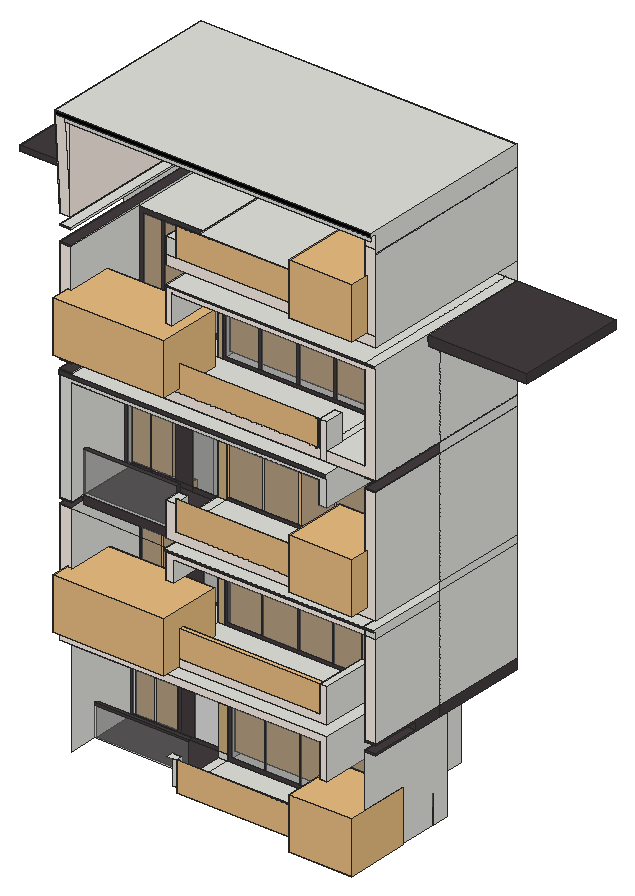
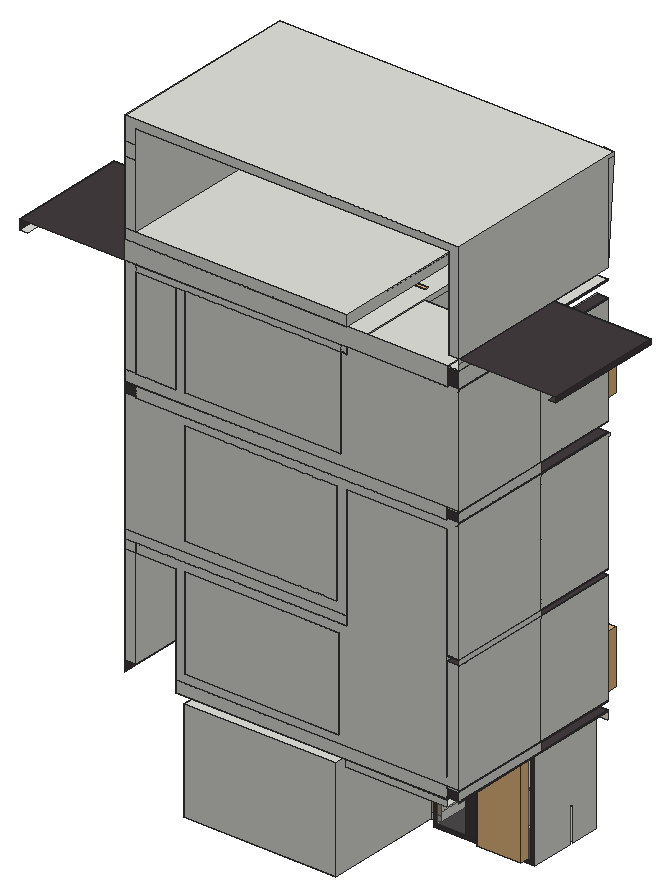
# SketchUp Ruby script. Lengths in inches.
U = 1.inch
M = Sketchup.active_model
def pt(a) = Geom::Point3d.new(a.map { |v| v * U })
def face(e, loops, mat)
  f = e.add_face(loops[0].map { |a| pt(a) })
  loops[1..].each { |l| e.add_face(l.map { |a| pt(a) }).erase! }
  f.material = f.back_material = mat if mat
  f
end
# faces: each face lists its corners as indices into pts; further lists are holes
def faces(e, pts, list, mat = nil) = list.each { |f| face(e, (f[0].is_a?(Array) ? f : [f]).map { |l| l.map { |i| pts[i] } }, mat) }
# xy, xz, yz: faces in a plane at the given z, y or x. An outline is a flat list of corners, or four numbers for a rectangle; further outlines are holes
def ring(l) = l.size == 4 ? [[l[0], l[1]], [l[2], l[1]], [l[2], l[3]], [l[0], l[3]]] : l.each_slice(2).to_a
def flat(e, list, mat, &to3) = list.each { |f| face(e, (f[0].is_a?(Array) ? f : [f]).map { |l| ring(l).map { |u, v| to3.(u, v) } }, mat) }
def xy(e, z, list, mat = nil) = flat(e, list, mat) { |x, y| [x, y, z] }
def xz(e, y, list, mat = nil) = flat(e, list, mat) { |x, z| [x, y, z] }
def yz(e, x, list, mat = nil) = flat(e, list, mat) { |y, z| [x, y, z] }
def lines(e, pts, list) = list.each { |a, b| e.add_line(pt(pts[a]), pt(pts[b])) }
# prism: a flat outline (further loops are holes) pulled along v
def prism(e, loops, v, mat = nil)
  f = face(e, loops, mat); d = Geom::Vector3d.new(v.map { |x| x * U })
  f.pushpull(f.normal.samedirection?(d) ? d.length : -d.length)
end
def box(e, o, s, mat = nil) = prism(e, [[o, [o[0] + s[0], o[1], o[2]], [o[0] + s[0], o[1] + s[1], o[2]], [o[0], o[1] + s[1], o[2]]]], [0, 0, s[2]], mat)
def at(x, y, z, deg = 0) = Geom::Transformation.translation(pt([x, y, z])) * Geom::Transformation.rotation(ORIGIN, Z_AXIS, deg.degrees)
def axes(o, x, y, z) = Geom::Transformation.new([*x, 0, *y, 0, *z, 0, *pt(o).to_a, 1])
def part(name) = M.definitions.add(name)
# library, detail: a bought-in or finely detailed component or shape, given as its bounding box
def library(name, o, s) = part(name).tap { |d| box(d.entities, o, s) }
def detail(e, o, s) = box(e.add_group.entities, o, s)
def put(e, d, t, mat = nil) = e.add_instance(d, t).tap { |i| i.material = mat if mat }
def group(e, t, mat = nil) = e.add_group.tap { |g| g.transformation = t; g.material = mat if mat }.entities
root = M.entities
M.materials.add("Material metal").color = [2, 2, 2]
M.materials.add("[0009_Linen]").color = [250, 240, 230]
M.materials.add("[Asphalt New]").color = [67, 60, 62]
M.materials.add("[Translucent Glass Gray]").color = [128, 128, 128]
M.materials["[Translucent Glass Gray]"].alpha = 0.5
M.materials.add("[Wood Floor Light]").color = [204, 176, 127]
c1 = library("Air Grill2",[0,0,0],[0.79,39.37,4.92])
c2 = library("Planted wooden trough",[0,0,0],[56.02,15.3,25.28])
c3 = library("fronceur+aubin+blanc+(3)",[-47.99,-0.29,1.66],[95.37,4.84,114.09])
xy(root,484.875,[[453.2,361.55,453.47,370.26],[453.47,361.55,628.99,361.55,628.99,440.43,453.2,440.43,453.2,370.26,453.47,370.26],[628.99,361.55,637.96,440.43],[637.96,361.55,684.21,463.55],[441.67,370.26,453.2,440.43],
  [453.2,440.43,628.99,577.24],[637.96,466.33,684.21,486.68]])
xy(root,484.875,[[325.03,399.42,441.42,450.18]],"[Asphalt New]")
xy(root,519.75,[[637.96,463.55,684.21,466.33]])
xy(root,520.45,[[441.67,361.55,453.2,370.26]])
xy(root,524.4375,[[325.03,394.93,441.42,399.42]],"[Asphalt New]")
xy(root,561.74,[[628.99,361.55,637.96,440.43]])
xy(root,602.15,[[325.03,361.55,325.03,519.74,325.23,519.74,325.23,577.24,441.67,577.24,441.67,440.43,628.99,440.43,628.99,361.55],[453.2,440.43,628.99,577.24]])
xy(root,609.74,[[325.03,450.18,441.42,577.24]])
xy(root,610.74,[[325.03,361.55,637.96,577.24]])
xy(root,610.74,[[637.96,422.24,684.21,486.68]],"[Asphalt New]")
xy(root,612.69,[[310.35,361.55,325.03,577.24]],"[Asphalt New]")
xy(root,612.78,[[684.21,361.55,697.64,422.24]],"[Asphalt New]")
xy(root,621.73,[[310.35,361.55,325.03,577.24]],"[Asphalt New]")
xy(root,622.21,[[684.21,361.55,697.64,422.24]],"[Asphalt New]")
xy(root,623.86,[[325.03,361.55,637.96,577.24],[637.96,422.24,637.96,428.24,684.21,428.24],[637.96,422.24,684.21,428.24,684.21,422.24]])
xy(root,623.86,[[637.96,428.24,684.21,486.68]],"[Asphalt New]")
xy(root,633.2,[[325.28,361.55,441.67,361.55,441.67,440.43,440.15,440.43,440.15,464.43,325.28,464.43],[441.67,361.55,449.31,375.68],[449.31,361.55,628.53,375.68],[441.67,375.68,628.53,440.43],[325.03,440.43,325.28,577.24],
  [449.31,440.43,628.53,577.24]])
xy(root,653.8,[[637.96,422.24,684.21,428.24]],"[Asphalt New]")
xy(root,665.58,[[628.53,361.55,637.96,425.8]])
xy(root,713.77,[[440.15,361.55,449.31,440.43]])
xy(root,739.02,[[449.31,361.55,449.31,440.43,628.53,440.43,628.53,425.8,637.96,425.8,637.96,486.68,684.21,486.68,684.21,361.55],[449.31,440.43,628.53,577.24],[637.96,486.68,684.21,577.24]])
xy(root,747.625,[[440.15,358.61,684.21,361.55],[684.21,358.61,697.64,361.55]],"[Asphalt New]")
xy(root,749.51,[[440.15,358.61,684.21,577.24],[684.21,358.61,697.64,577.24]])
xy(root,749.51,[[325.28,377.8,440.15,464.43]],"[Asphalt New]")
xy(root,753.26,[[310.35,361.55,325.28,577.24]],"[Asphalt New]")
xy(root,758.44,[[310.35,361.55,325.28,577.24]],"[Asphalt New]")
xy(root,759.64,[[440.15,361.55,684.21,577.24],[684.21,361.55,697.64,577.24],[325.28,377.8,440.15,382.77]])
xy(root,759.64,[[325.28,382.77,440.15,448.24]],"[Asphalt New]")
xy(root,765.32,[[325.28,440.43,329.77,448.24]],"[Asphalt New]")
xy(root,771.01,[[452.08,361.55,684.21,361.55,684.21,486.68,637.96,486.68,637.96,440.43,452.08,440.43],[440.15,380.85,452.08,440.43],[452.08,440.43,628.03,577.24]])
xy(root,802.1,[[440.15,361.55,452.08,380.85]])
xy(root,810.46,[[325.28,377.8,440.15,382.77]],"[Asphalt New]")
xy(root,862.01,[[628.03,361.55,637.96,440.43]])
xy(root,886.84,[[351.83,440.43,354,448.24],[382.72,440.43,404.17,448.24],[436.85,440.43,440.15,448.24]],"[Asphalt New]")
xy(root,886.84,[[329.77,440.43,351.83,448.24],[354,440.43,382.72,448.24],[404.17,440.43,436.85,448.24]],"[Translucent Glass Gray]")
xy(root,890.33,[[325.28,361.55,440.15,440.43],[440.15,361.55,452.08,440.43],[452.08,361.55,628.03,440.43],[452.08,440.43,628.03,577.24]])
xy(root,895.75,[[310.35,359.36,637.96,361.55]],"[Asphalt New]")
xy(root,899.82,[[325.28,359.36,637.96,577.24],[637.96,486.68,684.21,577.24]])
xy(root,899.82,[[310.35,359.36,325.28,361.55]],"[Asphalt New]")
xy(root,900.98,[[684.21,361.55,697.64,577.24]],"[Asphalt New]")
xy(root,901.48,[[310.35,361.55,325.28,577.24]],"[Asphalt New]")
xy(root,911.41,[[310.35,361.55,325.28,577.24]],"[Asphalt New]")
xy(root,911.67,[[684.21,361.55,697.64,577.24]],"[Asphalt New]")
xy(root,912.88,[[325.28,361.55,684.21,577.24]])
xy(root,924.85,[[323.4,361.55,628.53,361.55,628.53,440.43,325.28,440.43,325.28,465.68,323.4,465.68],[637.96,361.55,684.21,577.24],[628.53,384.47,637.96,440.43],[325.28,440.43,440.15,465.68],[447.28,440.43,628.53,577.24]])
xy(root,957.3,[[628.53,361.55,637.96,384.47]])
xy(root,995.8,[[440.15,361.55,447.28,440.43]])
xy(root,1027.125,[[697.64,440.82,818.95,458.82],[810.2,458.82,818.95,577.24]])
xy(root,1036.91,[[440.15,360.49,697.64,361.55]],"[Asphalt New]")
xy(root,1038.38,[[440.15,360.49,684.21,577.24],[684.21,360.49,697.64,577.24],[323.4,465.68,440.15,577.24]])
xy(root,1038.38,[[697.64,440.82,818.95,577.24]],"[Asphalt New]")
xy(root,1040.41,[[310.35,361.55,323.4,577.24]],"[Asphalt New]")
xy(root,1057.95,[[310.35,361.55,323.4,577.24]],"[Asphalt New]")
xy(root,1059.74,[[310.35,361.55,323.4,577.24],[440.15,361.55,684.21,577.24],[684.21,361.55,697.64,577.24]])
xy(root,1065.71,[[197.96,440.57,310.35,458.82],[197.96,458.82,206.14,577.24]],"[Asphalt New]")
xy(root,1071.68,[[310.35,361.55,322.68,577.24],[452.08,361.55,684.21,361.55,684.21,577.24,440.15,577.24,440.15,379.3,452.08,379.3],[439.45,379.3,440.15,577.24]])
xy(root,1071.68,[[197.96,440.57,310.35,577.24]],"[Asphalt New]")
xy(root,1092.06,[[440.15,361.55,452.08,379.3]])
xy(root,1178.92,[[322.68,361.55,684.21,577.24]],"[0009_Linen]")
xy(root,1184.18,[[310.35,352.99,697.64,361.55]],"Material metal")
xy(root,1188.32,[[310.35,352.99,697.64,577.24]])
xz(root,352.99,[[310.35,1184.18,697.64,1188.32]],"Material metal")
xz(root,358.61,[[440.15,747.625,684.21,749.51],[684.21,747.625,697.64,749.51]],"[Asphalt New]")
xz(root,359.36,[[310.35,895.75,637.96,899.82]],"[Asphalt New]")
xz(root,360.49,[[440.15,1036.91,697.64,1038.38]],"[Asphalt New]")
xz(root,361.55,[[684.21,739.02,697.64,747.625],[310.35,759.64,325.28,759.64,325.28,890.33,628.03,890.33,628.03,862.01,637.96,862.01,637.96,895.75,310.35,895.75],[440.15,1071.68,452.08,1092.06]])
xz(root,361.55,[[628.99,561.74,637.96,561.74,637.96,610.74,310.35,610.74,310.35,602.15,628.99,602.15],[310.35,623.86,637.96,623.86,637.96,665.58,628.53,665.58,628.53,633.2,325.28,633.2,325.28,751.61,310.35,751.89],[684.21,623.86,697.64,739.02],[440.15,713.77,449.31,713.77,449.31,739.02,684.21,739.02,684.21,747.625,440.15,747.625],[440.15,759.64,697.64,759.64,697.64,899.82,684.21,899.82,684.21,771.01,452.08,771.01,452.08,802.1,440.15,802.1],
  [310.35,912.88,628.53,912.88,628.53,924.85,323.4,924.85,323.4,1038.38,310.35,1038.38],[637.96,912.88,697.64,912.88,697.64,1036.91,440.15,1036.91,440.15,995.8,447.28,995.8,447.28,1030.55,684.21,1030.55,684.21,924.85,637.96,924.85],[628.53,912.88,637.96,957.3],[440.15,1059.74,697.64,1071.68],[310.35,1071.68,322.68,1071.68,322.68,1178.92,684.21,1178.92,684.21,1167.24,697.64,1167.24,697.64,1184.18,310.35,1184.18],
  [684.21,1071.68,697.64,1167.24]],"[0009_Linen]")
xz(root,361.55,[[310.35,610.74,325.03,612.69],[684.21,610.74,697.64,612.78],[310.35,621.73,325.03,623.86],[684.21,622.21,697.64,623.86],[325.28,751.61,325.28,753.26,310.35,753.26,310.35,751.89],
  [310.35,758.44,325.28,759.64],[310.35,899.82,325.28,901.48],[684.21,899.82,697.64,900.98],[310.35,911.41,325.28,912.88],[684.21,911.67,697.64,912.88],
  [310.35,1038.38,323.4,1040.41],[310.35,1057.95,323.4,1059.74]],"[Asphalt New]")
xz(root,370.26,[[441.67,484.875,453.2,520.45]])
xz(root,377.8,[[325.28,749.51,440.15,759.64]],"[Asphalt New]")
xz(root,377.8,[[325.28,759.64,440.15,810.46]],"[Translucent Glass Gray]")
xz(root,379.3,[[439.45,1071.68,440.15,1092.06],[440.15,1071.68,452.08,1092.06]])
xz(root,380.85,[[440.15,771.01,452.08,802.1]])
xz(root,384.47,[[628.53,924.85,637.96,957.3]])
xz(root,394.93,[[325.03,521.82,441.42,524.4375]],"[Asphalt New]")
xz(root,394.93,[[325.03,484.875,441.42,521.82]],"[Translucent Glass Gray]")
xz(root,422.24,[[637.96,610.74,684.21,623.86],[684.21,612.78,697.64,622.21],[637.96,652.52,684.21,653.8]],"[Asphalt New]")
xz(root,422.24,[[637.96,623.86,684.21,652.52]],"[Translucent Glass Gray]")
xz(root,425.8,[[628.53,665.58,637.96,739.02]],"[Wood Floor Light]")
xz(root,440.43,[[441.67,484.875,453.2,492.03],[325.28,890.33,440.15,924.85]])
xz(root,440.43,[[[453.2,484.875,628.99,602.15],[457.92,489.6,624.27,597.43]],[497.63,489.6,499.51,597.43],[541.09,489.6,542.98,597.43],[583.625,489.6,585.98,597.43],[[449.31,633.2,628.53,739.02],[452.58,636.47,625.26,735.75]],
  [494.64,636.47,495.75,735.75],[538.92,636.47,541.12,735.75],[581.8,636.47,583.1875,735.75],[325.28,765.32,329.77,886.84],[[452.08,771.01,628.03,890.33],[455.82,774.75,624.29,886.58]],
  [495.66,774.75,497.94,886.58],[540.06,774.75,543.15,886.58],[583.72,774.75,586,886.58],[325.28,886.84,351.83,890.33],[351.83,886.84,354,890.33],
  [354,886.84,382.72,890.33],[382.72,886.84,404.17,890.33],[404.17,886.84,436.85,890.33],[436.85,886.84,440.15,890.33],[[447.28,924.85,628.53,1030.55],[450.4,927.96,625.41,1027.43]],
  [491.4375,927.96,494.15,1027.43],[537.9,927.96,541.29,1027.43],[583.35,927.96,586.22,1027.43]],"[Asphalt New]")
xz(root,440.43,[[457.92,489.6,497.63,597.43],[499.51,489.6,541.09,597.43],[542.98,489.6,583.625,597.43],[585.98,489.6,624.27,597.43],[452.58,636.47,494.64,735.75],
  [495.75,636.47,538.92,735.75],[541.12,636.47,581.8,735.75],[583.1875,636.47,625.26,735.75],[455.82,774.75,495.66,886.58],[497.94,774.75,540.06,886.58],
  [543.15,774.75,583.72,886.58],[586,774.75,624.29,886.58],[450.4,927.96,491.4375,1027.43],[494.15,927.96,537.9,1027.43],[541.29,927.96,583.35,1027.43],
  [586.22,927.96,625.41,1027.43]],"[Translucent Glass Gray]")
xz(root,440.43,[[628.99,484.875,637.96,561.74],[441.67,492.03,453.2,602.15],[440.15,633.2,449.31,713.77],[440.15,771.01,452.08,890.33],[628.03,771.01,637.96,862.01],
  [440.15,924.85,447.28,995.8],[628.53,924.85,637.96,1030.55]],"[Wood Floor Light]")
xz(root,440.57,[[197.96,1065.71,310.35,1071.68]],"[Asphalt New]")
xz(root,440.82,[[697.64,1027.125,818.95,1038.38]],"[Asphalt New]")
xz(root,448.24,[[325.28,759.64,351.83,765.32],[351.83,759.64,354,765.32],[354,759.64,382.72,765.32],[382.72,759.64,404.17,765.32],[404.17,759.64,436.85,765.32],
  [436.85,759.64,440.15,765.32],[351.83,765.32,354,886.84],[382.72,765.32,404.17,886.84],[436.85,765.32,440.15,886.84]],"[Asphalt New]")
xz(root,448.24,[[329.77,765.32,351.83,886.84],[354,765.32,382.72,886.84],[404.17,765.32,436.85,886.84]],"[Translucent Glass Gray]")
xz(root,450.18,[[328.72,602.15,412.53,606.04]])
xz(root,450.18,[[[325.03,484.875,441.42,609.74],[328.72,488.57,437.72,606.04]],[355.97,488.57,358.23,602.15],[383.22,488.57,387.33,602.15],[387.33,488.57,404.66,602.15]],"[Asphalt New]")
xz(root,450.18,[[328.72,488.57,355.97,602.15],[358.23,488.57,383.22,602.15],[404.66,488.57,437.72,488.57,437.72,606.04,412.53,606.04,412.53,602.15,404.66,602.15]],"[Translucent Glass Gray]")
xz(root,463.55,[[637.96,518.16,684.21,519.75]],"[Asphalt New]")
xz(root,463.55,[[637.96,484.875,684.21,518.16]],"[Translucent Glass Gray]")
xz(root,464.43,[[[325.28,633.2,440.15,749.51],[328.21,636.13,437.22,746.58]],[352.86,636.13,355.46,746.58],[382.72,636.13,404.71,746.58]],"[Asphalt New]")
xz(root,464.43,[[328.21,636.13,352.86,746.58],[355.46,636.13,382.72,746.58],[404.71,636.13,437.22,746.58]],"[Translucent Glass Gray]")
xz(root,465.68,[[[323.4,924.85,440.15,1038.38],[329.24,930.68,434.32,1032.54]],[352.32,930.68,355.51,1032.54],[381.78,930.68,403.96,1032.54]],"[Asphalt New]")
xz(root,465.68,[[329.24,930.68,352.32,1032.54],[355.51,930.68,381.78,1032.54],[403.96,930.68,434.32,1032.54]],"[Translucent Glass Gray]")
xz(root,486.68,[[[637.96,484.875,684.21,610.74],[641.09,488.01,681.07,607.6]],[661.08,488.01,663.24,607.6],[[637.96,623.86,684.21,739.02],[640.79,626.69,681.37,736.18]],[661.08,626.69,662.58,736.18],[[637.96,771.01,684.21,899.82],[639.96,773.01,682.2,897.8125]],
  [661.08,773.01,663.38,897.8125]],"[Asphalt New]")
xz(root,486.68,[[641.09,488.01,661.08,607.6],[663.24,488.01,681.07,607.6],[640.79,626.69,661.08,736.18],[662.58,626.69,681.37,736.18],[639.96,773.01,661.08,897.8125],
  [663.38,773.01,682.2,897.8125]],"[Translucent Glass Gray]")
xz(root,577.24,[[453.2,484.875,628.99,602.15],[325.03,602.15,441.42,609.74],[325.03,610.74,637.96,623.86],[310.35,621.73,325.03,623.86],[[310.35,623.86,310.35,753.26,325.28,753.26,325.28,890.33,440.15,890.33,440.15,749.51,684.21,749.51,684.21,739.02,637.96,739.02,637.96,623.86],[449.31,633.2,628.53,739.02]],
  [684.21,623.86,697.64,739.02],[449.31,633.2,628.53,739.02],[684.21,739.02,697.64,749.51],[440.15,749.51,697.64,759.64],[310.35,758.44,325.28,759.64],
  [[310.35,759.64,310.35,901.48,325.28,901.48,325.28,899.82,684.21,899.82,684.21,900.98,697.64,900.98,697.64,759.64,440.15,759.64,440.15,890.33,325.28,890.33,325.28,759.64],[452.08,771.01,628.03,890.33]],[452.08,771.01,628.03,890.33],[325.28,899.82,684.21,912.88],[310.35,911.41,325.28,912.88],[684.21,911.67,697.64,912.88],
  [310.35,912.88,310.35,1040.41,323.4,1040.41,323.4,1038.38,440.15,1038.38,440.15,1030.55,447.28,1030.55,447.28,924.85,628.53,924.85,628.53,1030.55,637.96,1030.55,637.96,924.85,697.64,924.85,697.64,912.88],[447.28,924.85,628.53,1030.55],[637.96,924.85,684.21,1030.55],[684.21,924.85,697.64,1038.38],[440.15,1030.55,447.28,1031.85],
  [447.28,1030.55,684.21,1038.38],[440.15,1031.85,447.28,1038.38],[323.4,1038.38,697.64,1059.74],[310.35,1057.95,323.4,1059.74],[440.15,1059.74,697.64,1071.68],
  [310.35,1071.68,310.35,1188.32,697.64,1188.32,697.64,1162.16,684.21,1162.16,684.21,1178.92,322.68,1178.92,322.68,1071.68],[684.21,1071.68,697.64,1146.0625],[684.21,1146.0625,697.64,1162.16]])
xz(root,577.24,[[310.35,612.69,325.03,621.73],[684.21,900.98,697.64,911.67],[310.35,901.48,325.28,911.41],[310.35,1040.41,323.4,1057.95]],"[Asphalt New]")
yz(root,197.96,[[440.57,1065.71,577.24,1071.68]],"[Asphalt New]")
yz(root,310.35,[[458.82,612.69,577.24,621.73],[361.55,623.86,458.82,751.89],[458.82,623.86,577.24,751.89],[458.82,753.26,577.24,758.44],[361.55,759.64,361.55,895.75,359.36,895.75,359.36,899.82,458.82,899.82,458.82,759.64],
  [458.82,759.64,577.24,899.82],[458.82,901.48,577.24,911.41],[361.55,912.88,458.82,1038.38],[458.82,912.88,577.24,1038.38],[458.82,1040.41,577.24,1057.95],
  [458.82,1059.74,577.24,1065.71],[440.57,1065.71,577.24,1071.68],[361.55,1071.68,361.55,1184.18,353.29,1184.18,352.99,1188.32,577.24,1188.32,577.24,1071.68],[361.55,1071.68,353.29,1184.18,361.55,1184.18],[352.99,1184.18,352.99,1188.32,353.29,1184.18]])
yz(root,310.35,[[361.55,610.74,458.82,612.69],[458.82,610.74,577.24,612.69],[361.55,621.73,458.82,623.86],[458.82,621.73,577.24,623.86],[361.55,751.89,458.82,753.26],
  [458.82,751.89,577.24,753.26],[361.55,758.44,458.82,759.64],[458.82,758.44,577.24,759.64],[361.55,899.82,458.82,901.48],[458.82,899.82,577.24,901.48],
  [361.55,911.41,458.82,912.88],[458.82,911.41,577.24,912.88],[361.55,1038.38,458.82,1040.41],[458.82,1038.38,577.24,1040.41],[361.55,1057.95,458.82,1059.74],
  [458.82,1057.95,577.24,1059.74]],"[Asphalt New]")
yz(root,322.68,[[361.55,1071.68,577.24,1178.92]],"[0009_Linen]")
yz(root,323.4,[[361.55,924.85,465.68,1038.38],[361.55,1038.38,465.68,1040.41],[465.68,1038.38,577.24,1040.41],[361.55,1057.95,465.68,1059.74],[465.68,1057.95,577.24,1059.74]])
yz(root,325.03,[[361.55,484.875,394.93,484.875,394.93,524.4375,399.42,524.4375,399.42,484.875,450.18,484.875,450.18,602.15,361.55,602.15],[361.55,610.74,440.43,612.69],[440.43,610.74,577.24,612.69],[361.55,621.73,440.43,623.86],[440.43,621.73,577.24,623.86]])
yz(root,325.28,[[361.55,633.2,464.43,633.2,464.43,749.51,377.8,749.51,377.8,753.26,361.55,753.26],[464.43,633.2,577.24,753.26],[377.8,749.51,464.43,753.26],[377.8,753.26,464.43,758.44],[464.43,753.26,577.24,758.44],
  [361.55,758.44,377.8,759.64],[377.8,758.44,464.43,759.64],[464.43,758.44,577.24,759.64],[361.55,759.64,377.8,759.64,377.8,810.46,382.77,810.46,382.77,759.64,448.24,759.64,448.24,765.32,440.43,765.32,440.43,890.33,361.55,890.33],[448.24,759.64,577.24,759.64,577.24,890.33,440.43,890.33,440.43,765.32,448.24,765.32],
  [361.55,899.82,440.43,901.48],[440.43,899.82,577.24,901.48],[440.43,901.48,577.24,911.41],[361.55,911.41,440.43,912.88],[440.43,911.41,577.24,912.88]])
yz(root,325.28,[[377.8,759.64,382.77,810.46]],"[Asphalt New]")
yz(root,329.77,[[440.43,765.32,448.24,886.84]],"[Translucent Glass Gray]")
yz(root,440.15,[[361.55,713.77,361.55,747.625,358.61,747.625,358.61,749.51,464.43,749.51,464.43,713.77],[377.8,749.51,577.24,759.64],[361.55,759.64,377.8,802.1],[377.8,759.64,377.8,802.1,380.85,802.1,380.85,771.01,382.77,771.01,382.77,759.64],[382.77,759.64,448.24,771.01],
  [448.24,759.64,448.24,886.84,440.43,886.84,440.43,890.33,577.24,890.33,577.24,759.64],[440.43,924.85,465.68,995.8],[361.55,995.8,465.68,1031.85],[465.68,1030.55,577.24,1031.85],[361.55,1031.85,361.55,1036.91,360.49,1036.91,360.49,1038.38,465.68,1038.38,465.68,1031.85],
  [465.68,1031.85,577.24,1038.38],[361.55,1059.74,361.55,1092.06,379.3,1092.06,379.3,1071.68,577.24,1071.68,577.24,1059.74]])
yz(root,440.15,[[440.43,633.2,464.43,713.77],[380.85,771.01,382.77,771.01,382.77,810.46,377.8,810.46,377.8,802.1,380.85,802.1],[440.43,771.01,448.24,859.69],[440.43,859.69,448.24,886.84]],"[Asphalt New]")
yz(root,447.28,[[440.43,924.85,577.24,924.85,577.24,1031.85,361.55,1031.85,361.55,995.8,440.43,995.8]])
yz(root,449.31,[[440.43,633.2,577.24,739.02],[361.55,713.77,440.43,739.02]])
yz(root,452.08,[[361.55,771.01,380.85,802.1],[440.43,771.01,577.24,890.33],[361.55,1071.68,379.3,1092.06]])
yz(root,453.2,[[361.55,484.875,370.26,520.45],[440.43,484.875,577.24,602.15]])
yz(root,628.03,[[440.43,771.01,577.24,890.33],[361.55,862.01,440.43,890.33]])
yz(root,628.53,[[361.55,633.2,361.55,665.58,425.8,665.58,425.8,739.02,440.43,739.02,440.43,633.2],[440.43,633.2,577.24,739.02],[361.55,924.85,384.47,957.3],[440.43,924.85,577.24,1030.55]])
yz(root,628.99,[[440.43,484.875,577.24,602.15],[361.55,561.74,440.43,602.15]])
yz(root,637.96,[[440.43,484.875,463.55,484.875,463.55,519.75,466.33,519.75,466.33,484.875,486.68,484.875,486.68,610.74,440.43,610.74],[361.55,561.74,440.43,610.74],[422.24,610.74,577.24,623.86],[361.55,623.86,422.24,623.86,422.24,653.8,428.24,653.8,428.24,623.86,440.43,623.86,440.43,739.02,425.8,739.02,425.8,665.58,361.55,665.58],[440.43,623.86,486.68,739.02],
  [486.68,623.86,577.24,739.02],[440.43,771.01,486.68,771.01,486.68,899.82,359.36,899.82,359.36,895.75,361.55,895.75,361.55,862.01,440.43,862.01],[361.55,924.85,384.47,957.3],[440.43,924.85,577.24,1030.55]])
yz(root,637.96,[[422.24,623.86,428.24,653.8]],"[Asphalt New]")
yz(root,684.21,[[361.55,484.875,361.55,610.74,486.68,610.74,486.68,484.875,466.33,484.875,466.33,519.75,463.55,519.75,463.55,484.875],[422.24,610.74,486.68,623.86],[361.55,623.86,361.55,739.02,486.68,739.02,486.68,623.86,428.24,623.86,428.24,653.8,422.24,653.8,422.24,623.86],[486.68,623.86,577.24,739.02],[361.55,739.02,361.55,747.625,358.61,747.625,358.61,749.51,577.24,749.51,577.24,739.02],
  [361.55,771.01,486.68,899.82],[486.68,899.82,577.24,900.98],[486.68,911.67,577.24,912.88],[361.55,924.85,577.24,1030.55],[361.55,1071.68,577.24,1178.92]])
yz(root,684.21,[[361.55,610.74,422.24,612.78],[361.55,622.21,422.24,623.86],[422.24,623.86,428.24,653.8],[361.55,899.82,486.68,900.98],[361.55,911.67,486.68,912.88]],"[Asphalt New]")
yz(root,697.64,[[361.55,623.86,458.82,739.02],[458.82,623.86,577.24,749.51],[361.55,739.02,458.82,739.02,458.82,749.51,358.61,749.51,358.61,747.625,361.55,747.625],[458.82,749.51,577.24,759.64],[361.55,759.64,458.82,899.82],
  [458.82,759.64,577.24,899.82],[458.82,900.98,577.24,911.67],[361.55,912.88,458.82,912.88,458.82,1027.125,440.82,1027.125,440.82,1038.38,360.49,1038.38,360.49,1036.91,361.55,1036.91],[458.82,912.88,458.82,1027.125,440.82,1027.125,440.82,1038.38,577.24,1038.38,577.24,912.88],[361.55,1059.74,577.24,1161.875],
  [361.55,1161.875,577.24,1162.16],[361.55,1162.16,577.24,1162.18],[361.55,1162.18,577.24,1162.18,577.24,1188.32,352.99,1188.32,352.99,1184.18,361.55,1184.18]])
yz(root,697.64,[[361.55,610.74,458.82,610.74,458.82,623.86,361.55,623.86,361.55,622.21,422.24,622.21,422.24,612.78,361.55,612.78],[458.82,610.74,577.24,623.86],[361.55,899.82,458.82,900.98],[458.82,899.82,577.24,900.98],[361.55,911.67,458.82,912.88],
  [458.82,911.67,577.24,912.88]],"[Asphalt New]")
yz(root,818.95,[[440.82,1027.125,577.24,1038.38]],"[Asphalt New]")
p = [[310.35,352.99,1188.32],[310.35,353.29,1184.18],[310.35,361.55,1071.68],[322.68,361.55,1071.68],[322.68,353.64,1179.45],[322.68,353.29,1184.2],
  [322.68,352.99,1188.32],[697.64,353.34,1179.43],[697.64,352.99,1184.18],[637.96,361.55,912.87],[637.96,361.55,912.88],[452.08,380.85,1071.68],
  [452.08,379.3,1071.68],[684.21,577.24,1038.38],[684.21,577.24,1039.57],[325.03,440.43,609.74],[325.03,440.43,610.74],[637.96,486.68,739.02],
  [637.96,486.68,771.01],[325.03,440.43,623.86],[325.03,440.43,633.2],[440.15,361.55,749.51],[325.28,361.55,751.61],[310.35,577.24,899.82],
  [310.35,582.18,899.82],[310.35,577.24,1038.38],[310.35,579.68,1038.38]]
faces(root,p,[[0,1,2,3,4,5,6]],"[0009_Linen]")
faces(root,p,[[7,8,5,4]])
lines(root,p,[[9,10],[11,12],[13,14],[15,16],[17,18],[19,20],[21,22],[23,24],[25,26]])
put(root,c1,axes([453.24,361.55,484.46],[0,0.7772,0],[3.99656,0,0],[0,0,7.31206]))
put(root,c2,axes([609.09,338.71,484.875],[1.3851,0,0],[0,5.103,0],[0,0,2.4786]))
put(root,c3,axes([357.95,450.81,488.39],[0.53351,0,0],[0,2.19308,0],[0,0,0.98284]))
put(root,c3,axes([542.94,449.8125,493.55],[1.7888,0,0],[0,-1,0],[0,0,0.92721]))
put(root,c2,axes([319.25,338.82,623.86],[2.43,0,0],[0,5.103,0],[0,0,2.4786]))
put(root,c1,axes([448.09,361.66,632.79],[0,8.4082,0],[4.58502,0,0],[0,0,6.67858]))
put(root,c3,axes([537.6,449.8125,631.87],[1.7888,0,0],[0,-1,0],[0,0,0.92721]))
put(root,c3,axes([354.24,483.7,635.03],[0.53351,0,0],[0,-4.23732,0],[0,0,0.98284]))
put(root,c3,axes([354.24,453.4,766.13],[0.53351,0,0],[0,-1.13546,0],[0,0,1.05164]))
put(root,c2,axes([609.09,338.71,769.67],[1.3851,0,0],[0,5.103,0],[0,0,2.4786]))
put(root,c1,axes([451.85,361.55,770.72],[0,0.7772,0],[4.03196,0,0],[0,0,7.31206]))
put(root,c3,axes([537.6,440.71,773.05],[1.7888,0,0],[0,1,0],[0,0,1.02185]))
put(root,c3,axes([354.36,471.63,921.31],[0.53351,0,0],[0,-1.13546,0],[0,0,0.98284]))
put(root,c1,axes([448.09,361.55,924.43],[0,0.141,0],[4.53738,0,0],[0,0,6.67858]))
put(root,c2,axes([319.25,338.82,928.85],[2.43,0,0],[0,5.103,0],[0,0,2.4786]))
put(root,c3,axes([537.6,449.8125,931.06],[1.7888,0,0],[0,-1,0],[0,0,0.92721]))
put(root,c1,axes([451.85,361.55,1071.39],[0,0.7772,0],[5.86763,0,0],[0,0,7.31206]))
put(root,c2,axes([609.09,338.71,1071.68],[1.3851,0,0],[0,5.103,0],[0,0,2.4786]))
